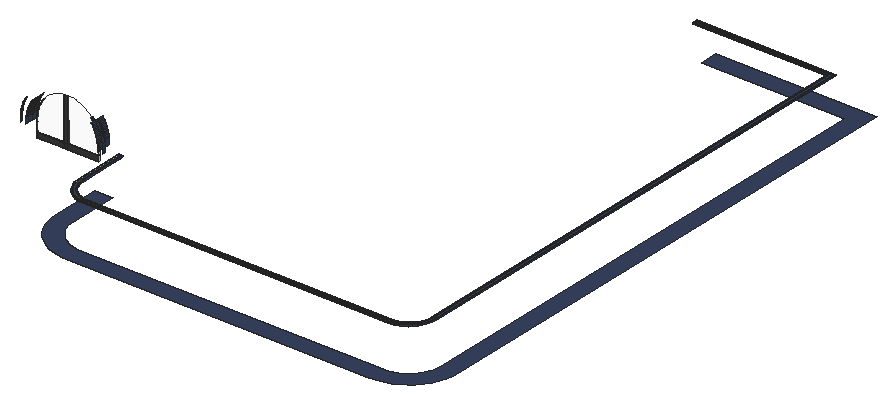
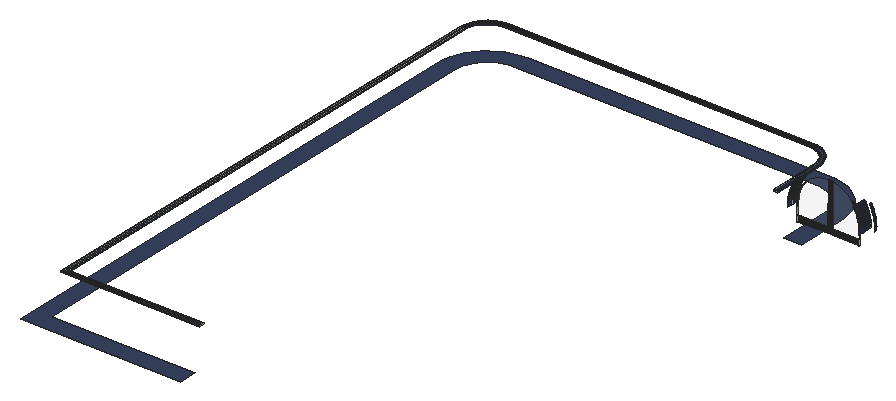
# SketchUp Ruby script. Lengths in inches.
U = 1.inch
M = Sketchup.active_model
def pt(a) = Geom::Point3d.new(a.map { |v| v * U })
def face(e, loops, mat)
  f = e.add_face(loops[0].map { |a| pt(a) })
  loops[1..].each { |l| e.add_face(l.map { |a| pt(a) }).erase! }
  f.material = f.back_material = mat if mat
  f
end
# faces: each face lists its corners as indices into pts; further lists are holes
def faces(e, pts, list, mat = nil) = list.each { |f| face(e, (f[0].is_a?(Array) ? f : [f]).map { |l| l.map { |i| pts[i] } }, mat) }
# xy, xz, yz: faces in a plane at the given z, y or x. An outline is a flat list of corners, or four numbers for a rectangle; further outlines are holes
def ring(l) = l.size == 4 ? [[l[0], l[1]], [l[2], l[1]], [l[2], l[3]], [l[0], l[3]]] : l.each_slice(2).to_a
def flat(e, list, mat, &to3) = list.each { |f| face(e, (f[0].is_a?(Array) ? f : [f]).map { |l| ring(l).map { |u, v| to3.(u, v) } }, mat) }
def xy(e, z, list, mat = nil) = flat(e, list, mat) { |x, y| [x, y, z] }
def xz(e, y, list, mat = nil) = flat(e, list, mat) { |x, z| [x, y, z] }
def yz(e, x, list, mat = nil) = flat(e, list, mat) { |y, z| [x, y, z] }
def lines(e, pts, list) = list.each { |a, b| e.add_line(pt(pts[a]), pt(pts[b])) }
# prism: a flat outline (further loops are holes) pulled along v
def prism(e, loops, v, mat = nil)
  f = face(e, loops, mat); d = Geom::Vector3d.new(v.map { |x| x * U })
  f.pushpull(f.normal.samedirection?(d) ? d.length : -d.length)
end
def box(e, o, s, mat = nil) = prism(e, [[o, [o[0] + s[0], o[1], o[2]], [o[0] + s[0], o[1] + s[1], o[2]], [o[0], o[1] + s[1], o[2]]]], [0, 0, s[2]], mat)
def at(x, y, z, deg = 0) = Geom::Transformation.translation(pt([x, y, z])) * Geom::Transformation.rotation(ORIGIN, Z_AXIS, deg.degrees)
def axes(o, x, y, z) = Geom::Transformation.new([*x, 0, *y, 0, *z, 0, *pt(o).to_a, 1])
def part(name) = M.definitions.add(name)
# library, detail: a bought-in or finely detailed component or shape, given as its bounding box
def library(name, o, s) = part(name).tap { |d| box(d.entities, o, s) }
def detail(e, o, s) = box(e.add_group.entities, o, s)
def put(e, d, t, mat = nil) = e.add_instance(d, t).tap { |i| i.material = mat if mat }
def group(e, t, mat = nil) = e.add_group.tap { |g| g.transformation = t; g.material = mat if mat }.entities
root = M.entities
M.materials.add("0360 AP 9644 Monsoon Midnight-N").color = [56, 67, 95]
M.materials.add("Glass Clear 001").color = [246, 246, 246]
M.materials["Glass Clear 001"].alpha = 0.1
M.materials.add("[Color M07]").color = [58, 58, 58]
xy(root,273.625,[[134.21,17.08,360,17.08,364.8125,17.39,369.54,18.34,374.11,19.88,378.43,22.02,382.4375,24.7,386.0625,27.875,389.24,31.5,391.92,35.51,394.05,39.83,395.6,44.4,396.54,49.125,396.86,53.9375,396.86,438.8,278.3125,438.8,278.3125,425.9375,384,425.9375,384,53.9375,383.79,50.8,383.18,47.73,382.17,44.75,380.78,41.9375,379.04,39.33,376.97,36.97,374.61,34.9,372,33.15,369.18,31.76,366.21,30.76,363.13,30.14,360,29.9375,134.95,29.9375,131.9375,30.29,128.99,31.02,126.8125,31.86,126.15,32.11,123.48,33.56,121.01,35.33,118.78,37.4,116.84,39.73,115.2,42.29,113.9,45.03,112.95,47.92,112.38,50.91,112.1875,53.9375,112.1875,89.9375,99.33,89.9375,99.33,53.53,99.6,49.28,100.48,44.7,101.93,40.26,103.93,36.04,106.45,32.11,109.4375,28.53,112.86,25.35,116.65,22.63,120.76,20.42,122.17,19.87,125.11,18.73,129.64,17.61]],"0360 AP 9644 Monsoon Midnight-N")
xy(root,291.19,[[53.24,93.58,73.03,94.27],[76.4,93.58,98.89,94.27]])
xy(root,294.87,[[53.24,93.58,73.03,94.27],[76.36,93.58,98.89,94.27]],"[Color M07]")
xy(root,302.6875,[[135.22,34.55,132.76,34.83,130.375,35.42,128.47,36.16,128.09,36.31,125.93,37.47,123.93,38.9,122.13,40.57,120.5625,42.46,119.24,44.53,118.1875,46.74,117.42,49.08,116.96,51.49,116.8,54.08,116.8,89.9375,118.94,89.9375,118.94,54.15,119.09,51.76,119.5,49.62,120.18,47.54,121.12,45.57,122.29,43.73,123.69,42.05,125.29,40.57,127.07,39.3,128.99,38.26,129.25,38.16,131.02,37.47,133.14,36.95,135.35,36.69,360,36.69,362.25,36.84,364.46,37.28,366.6,38,368.625,39,370.5,40.25,372.2,41.74,373.68,43.4375,374.9375,45.3125,375.93,47.34,376.66,49.47,377.1,51.6875,377.25,53.9375,377.25,419.18,278.3125,419.18,278.3125,421.33,379.39,421.33,379.39,53.9375,379.23,51.41,378.73,48.92,377.92,46.52,376.79,44.24,375.39,42.13,373.71,40.23,371.81,38.55,369.7,37.14,367.42,36.02,365.02,35.21,362.53,34.71,360,34.55]])
xy(root,302.6875,[[[135.18,33.89,132.64,34.18,130.18,34.79,128.24,35.54,127.8125,35.71,125.58,36.92,123.52,38.39,121.66,40.12,120.03,42.07,118.66,44.21,117.58,46.5,116.79,48.91,116.31,51.4,116.14,54.0625,116.14,90.59,119.6,90.59,119.6,54.17,119.74,51.84,120.14,49.78,120.79,47.78,121.69,45.89,122.83,44.12,124.17,42.51,125.71,41.08,127.42,39.85,129.26,38.86,129.48,38.77,131.22,38.1,133.26,37.59,135.38,37.35,360,37.35,362.17,37.49,364.29,37.91,366.35,38.61,368.3,39.57,370.1,40.78,371.73,42.21,373.16,43.84,374.37,45.64,375.33,47.59,376.03,49.64,376.45,51.77,376.59,53.9375,376.59,418.53,277.66,418.53,277.66,421.99,380.05,421.99,380.05,53.9375,379.88,51.32,379.37,48.75,378.52,46.27,377.36,43.91,375.91,41.73,374.18,39.76,372.2,38.03,370.02,36.57,367.67,35.42,365.1875,34.57,362.62,34.06,360,33.89],[135.22,34.55,360,34.55,362.53,34.71,365.02,35.21,367.42,36.02,369.7,37.14,371.81,38.55,373.71,40.23,375.39,42.13,376.79,44.24,377.92,46.52,378.73,48.92,379.23,51.41,379.39,53.9375,379.39,421.33,278.3125,421.33,278.3125,419.18,377.25,419.18,377.25,53.9375,377.1,51.6875,376.66,49.47,375.93,47.34,374.9375,45.3125,373.68,43.4375,372.2,41.74,370.5,40.25,368.625,39,366.6,38,364.46,37.28,362.25,36.84,360,36.69,135.35,36.69,133.14,36.95,131.02,37.47,129.25,38.16,128.99,38.26,127.07,39.3,125.29,40.57,123.69,42.05,122.29,43.73,121.12,45.57,120.18,47.54,119.5,49.62,119.09,51.76,118.94,54.15,118.94,89.9375,116.8,89.9375,116.8,54.08,116.96,51.49,117.42,49.08,118.1875,46.74,119.24,44.53,120.5625,42.46,122.13,40.57,123.93,38.9,125.93,37.47,128.09,36.31,128.47,36.16,130.375,35.42,132.76,34.83]]],"0360 AP 9644 Monsoon Midnight-N")
xy(root,303.4375,[[[135.18,33.89,360,33.89,362.62,34.06,365.1875,34.57,367.67,35.42,370.02,36.57,372.2,38.03,374.18,39.76,375.91,41.73,377.36,43.91,378.52,46.27,379.37,48.75,379.88,51.32,380.05,53.9375,380.05,421.99,277.66,421.99,277.66,418.53,376.59,418.53,376.59,53.9375,376.45,51.77,376.03,49.64,375.33,47.59,374.37,45.64,373.16,43.84,371.73,42.21,370.1,40.78,368.3,39.57,366.35,38.61,364.29,37.91,362.17,37.49,360,37.35,135.38,37.35,133.26,37.59,131.22,38.1,129.48,38.77,129.26,38.86,127.42,39.85,125.71,41.08,124.17,42.51,122.83,44.12,121.69,45.89,120.79,47.78,120.14,49.78,119.74,51.84,119.6,54.17,119.6,90.59,116.14,90.59,116.14,54.0625,116.31,51.4,116.79,48.91,117.58,46.5,118.66,44.21,120.03,42.07,121.66,40.12,123.52,38.39,125.58,36.92,127.8125,35.71,128.24,35.54,130.18,34.79,132.64,34.18],[135.22,34.55,132.76,34.83,130.375,35.42,128.47,36.16,128.09,36.31,125.93,37.47,123.93,38.9,122.13,40.57,120.5625,42.46,119.24,44.53,118.1875,46.74,117.42,49.08,116.96,51.49,116.8,54.08,116.8,89.9375,118.94,89.9375,118.94,54.15,119.09,51.76,119.5,49.62,120.18,47.54,121.12,45.57,122.29,43.73,123.69,42.05,125.29,40.57,127.07,39.3,128.99,38.26,129.25,38.16,131.02,37.47,133.14,36.95,135.35,36.69,360,36.69,362.25,36.84,364.46,37.28,366.6,38,368.625,39,370.5,40.25,372.2,41.74,373.68,43.4375,374.9375,45.3125,375.93,47.34,376.66,49.47,377.1,51.6875,377.25,53.9375,377.25,419.18,278.3125,419.18,278.3125,421.33,379.39,421.33,379.39,53.9375,379.23,51.41,378.73,48.92,377.92,46.52,376.79,44.24,375.39,42.13,373.71,40.23,371.81,38.55,369.7,37.14,367.42,36.02,365.02,35.21,362.53,34.71,360,34.55]],[135.22,34.55,360,34.55,362.53,34.71,365.02,35.21,367.42,36.02,369.7,37.14,371.81,38.55,373.71,40.23,375.39,42.13,376.79,44.24,377.92,46.52,378.73,48.92,379.23,51.41,379.39,53.9375,379.39,421.33,278.3125,421.33,278.3125,419.18,377.25,419.18,377.25,53.9375,377.1,51.6875,376.66,49.47,375.93,47.34,374.9375,45.3125,373.68,43.4375,372.2,41.74,370.5,40.25,368.625,39,366.6,38,364.46,37.28,362.25,36.84,360,36.69,135.35,36.69,133.14,36.95,131.02,37.47,129.25,38.16,128.99,38.26,127.07,39.3,125.29,40.57,123.69,42.05,122.29,43.73,121.12,45.57,120.18,47.54,119.5,49.62,119.09,51.76,118.94,54.15,118.94,89.9375,116.8,89.9375,116.8,54.08,116.96,51.49,117.42,49.08,118.1875,46.74,119.24,44.53,120.5625,42.46,122.13,40.57,123.93,38.9,125.93,37.47,128.09,36.31,128.47,36.16,130.375,35.42,132.76,34.83]],"0360 AP 9644 Monsoon Midnight-N")
xz(root,33.89,[[135.18,302.6875,360,303.4375]],"0360 AP 9644 Monsoon Midnight-N")
xz(root,34.55,[[135.22,302.6875,360,303.4375]])
xz(root,36.69,[[135.35,302.6875,360,303.4375]])
xz(root,37.35,[[135.38,302.6875,360,303.4375]],"0360 AP 9644 Monsoon Midnight-N")
xz(root,89.9375,[[49.72,301.29,49.72,305.77,49.71,305.66,49.65,304.79,49.625,303.91,49.63,303.04,49.66,302.16],[102.41,301.29,102.47,302.16,102.5,303.04,102.5,303.91,102.47,304.79,102.42,305.66,102.41,305.77],[116.8,302.6875,117.8125,303.4375],[117.8125,302.6875,118.94,303.4375]])
xz(root,90.59,[[116.14,302.6875,117.8125,303.4375],[117.8125,302.6875,119.6,303.4375]])
xz(root,93.58,[[53.24,291.19,73.03,294.87],[73.03,291.19,76.4,291.19,76.36,294.87,73.03,294.87],[76.4,291.19,98.89,291.19,98.89,294.87,76.36,294.87],[73.03,294.87,76.36,294.87,76.0625,326.46,75.3,326.45,74.55,326.41,73.79,326.35,73.03,326.26]],"[Color M07]")
xz(root,94.27,[[53.24,294.87,73.03,294.87,73.03,326.26,72.28,326.15,71.54,326.01,70.8,325.85,70.06,325.66,69.33,325.45,68.61,325.21,67.9,324.95,67.19,324.67,66.5,324.37,65.8125,324.04,65.14,323.6875,64.48,323.32,63.83,322.92,63.19,322.51,62.57,322.07,61.97,321.61,61.375,321.13,60.8,320.64,60.24,320.125,59.7,319.59,59.18,319.04,58.67,318.47,58.19,317.89,57.72,317.29,57.28,316.67,56.85,316.05,56.45,315.4,56.07,314.75,55.71,314.08,55.37,313.4,55.06,312.71,54.76,312.01,54.49,311.3,54.25,310.58,54.03,309.85,53.83,309.12,53.66,308.38,53.51,307.64,53.39,306.89,53.29,306.13,53.24,305.6],[76.36,294.87,98.89,294.87,98.89,305.6,98.84,306.13,98.74,306.89,98.62,307.64,98.47,308.38,98.29,309.12,98.1,309.85,97.875,310.58,97.63,311.3,97.36,312.01,97.07,312.71,96.75,313.4,96.42,314.08,96.06,314.75,95.67,315.4,95.27,316.05,94.85,316.67,94.4,317.29,93.94,317.89,93.45,318.47,92.95,319.04,92.42,319.59,91.88,320.125,91.32,320.64,90.75,321.13,90.16,321.61,89.55,322.07,88.93,322.51,88.3,322.92,87.65,323.32,86.99,323.6875,86.3125,324.04,85.63,324.37,84.93,324.67,84.23,324.95,83.52,325.21,82.79,325.45,82.06,325.66,81.33,325.85,80.59,326.01,79.84,326.15,79.09,326.26,78.34,326.35,77.58,326.41,76.82,326.45,76.0625,326.46]],"Glass Clear 001")
xz(root,418.53,[[277.66,302.6875,376.59,303.4375]])
xz(root,419.18,[[278.3125,302.6875,377.25,303.4375]])
xz(root,421.33,[[278.3125,302.6875,379.39,303.4375]])
xz(root,421.99,[[277.66,302.6875,380.05,303.4375]])
yz(root,49.72,[[88.375,301.29,89.9375,305.77],[89.9375,301.29,93.58,305.77],[94.96,301.29,98.79,305.77]],"0360 AP 9644 Monsoon Midnight-N")
yz(root,49.72,[[93.58,301.29,94.96,305.77]],"[Color M07]")
yz(root,53.24,[[93.58,291.19,94.96,294.87]])
yz(root,53.24,[[93.58,294.87,94.27,301.29],[93.58,301.29,94.27,305.6]],"[Color M07]")
yz(root,73.03,[[93.58,294.87,94.27,326.26]],"[Color M07]")
yz(root,98.89,[[93.58,291.19,94.96,294.87],[94.27,294.87,94.96,301.29],[94.27,301.29,94.96,305.6]])
yz(root,98.89,[[93.58,294.87,94.27,301.29],[93.58,301.29,94.27,305.6]],"[Color M07]")
yz(root,102.41,[[93.58,301.29,94.96,305.77]])
yz(root,102.41,[[88.375,301.29,89.9375,305.77],[89.9375,301.29,93.58,305.77],[94.96,301.29,98.79,305.77]],"0360 AP 9644 Monsoon Midnight-N")
yz(root,102.5,[[88.375,303.04,89.9375,303.91]])
yz(root,116.14,[[54.0625,302.6875,90.59,303.4375]],"0360 AP 9644 Monsoon Midnight-N")
yz(root,116.8,[[54.08,302.6875,89.9375,303.4375]])
yz(root,118.94,[[54.15,302.6875,89.9375,303.4375]])
yz(root,119.6,[[54.17,302.6875,90.59,303.4375]],"0360 AP 9644 Monsoon Midnight-N")
yz(root,277.66,[[418.53,302.6875,421.99,303.4375]])
yz(root,278.3125,[[419.18,302.6875,421.33,303.4375]])
yz(root,376.59,[[53.9375,302.6875,418.53,303.4375]],"0360 AP 9644 Monsoon Midnight-N")
yz(root,377.25,[[53.9375,302.6875,419.18,303.4375]])
yz(root,379.39,[[53.9375,302.6875,421.33,303.4375]])
yz(root,380.05,[[53.9375,302.6875,421.99,303.4375]],"0360 AP 9644 Monsoon Midnight-N")
p = [[76.36,94.27,294.87],[76.0625,94.27,326.46],[76.0625,93.58,326.46],[76.36,93.58,294.87],[45.48,89.9375,301.94],[45.54,89.9375,301.15],
  [45.54,88.375,301.15],[45.48,88.375,301.94],[106.59,89.9375,301.15],[106.64,89.9375,301.94],[106.64,88.375,301.94],[106.59,88.375,301.15],
  [49.72,89.9375,301.29],[49.66,89.9375,302.16],[49.66,88.375,302.16],[49.72,88.375,301.29],[102.47,89.9375,302.16],[102.41,89.9375,301.29],
  [102.41,88.375,301.29],[102.47,88.375,302.16],[45.45,89.9375,302.96],[45.45,88.375,302.96],[106.63,89.9375,304.01],[106.63,88.375,304.01],
  [49.63,89.9375,303.04],[49.63,88.375,303.04],[102.5,89.9375,303.04],[102.5,88.375,303.04],[132.64,34.18,302.6875],[135.18,33.89,302.6875],
  [135.18,33.89,303.4375],[132.64,34.18,303.4375],[360,33.89,302.6875],[362.62,34.06,302.6875],[362.62,34.06,303.4375],[360,33.89,303.4375],
  [365.1875,34.57,302.6875],[365.1875,34.57,303.4375],[130.18,34.79,302.6875],[130.18,34.79,303.4375],[135.22,34.55,302.6875],[132.76,34.83,302.6875],
  [132.76,34.83,303.4375],[135.22,34.55,303.4375],[362.53,34.71,302.6875],[360,34.55,302.6875],[360,34.55,303.4375],[362.53,34.71,303.4375],
  [367.67,35.42,302.6875],[367.67,35.42,303.4375],[365.02,35.21,302.6875],[365.02,35.21,303.4375],[128.24,35.54,302.6875],[128.24,35.54,303.4375],
  [130.375,35.42,302.6875],[130.375,35.42,303.4375],[367.42,36.02,302.6875],[367.42,36.02,303.4375],[128.47,36.16,302.6875],[128.47,36.16,303.4375],
  [370.02,36.57,302.6875],[370.02,36.57,303.4375],[127.8125,35.71,302.6875],[127.8125,35.71,303.4375],[125.58,36.92,302.6875],[125.58,36.92,303.4375],
  [369.7,37.14,302.6875],[369.7,37.14,303.4375],[128.09,36.31,302.6875],[128.09,36.31,303.4375],[125.93,37.47,302.6875],[125.93,37.47,303.4375],
  [372.2,38.03,302.6875],[372.2,38.03,303.4375],[133.14,36.95,302.6875],[135.35,36.69,302.6875],[135.35,36.69,303.4375],[133.14,36.95,303.4375],
  [360,36.69,302.6875],[362.25,36.84,302.6875],[362.25,36.84,303.4375],[360,36.69,303.4375],[364.46,37.28,302.6875],[364.46,37.28,303.4375],
  [123.52,38.39,302.6875],[123.52,38.39,303.4375],[131.02,37.47,302.6875],[131.02,37.47,303.4375],[371.81,38.55,302.6875],[371.81,38.55,303.4375],
  [135.38,37.35,302.6875],[133.26,37.59,302.6875],[133.26,37.59,303.4375],[135.38,37.35,303.4375],[362.17,37.49,302.6875],[360,37.35,302.6875],
  [360,37.35,303.4375],[362.17,37.49,303.4375],[366.6,38,302.6875],[366.6,38,303.4375],[123.93,38.9,302.6875],[123.93,38.9,303.4375],
  [129.25,38.16,302.6875],[129.25,38.16,303.4375],[364.29,37.91,302.6875],[364.29,37.91,303.4375],[131.22,38.1,302.6875],[131.22,38.1,303.4375],
  [366.35,38.61,302.6875],[366.35,38.61,303.4375],[368.625,39,302.6875],[368.625,39,303.4375],[374.18,39.76,302.6875],[374.18,39.76,303.4375],
  [129.48,38.77,302.6875],[129.48,38.77,303.4375],[128.99,38.26,302.6875],[128.99,38.26,303.4375],[127.07,39.3,302.6875],[127.07,39.3,303.4375],
  [121.66,40.12,302.6875],[121.66,40.12,303.4375],[368.3,39.57,302.6875],[368.3,39.57,303.4375],[373.71,40.23,302.6875],[373.71,40.23,303.4375],
  [129.26,38.86,302.6875],[129.26,38.86,303.4375],[122.13,40.57,302.6875],[122.13,40.57,303.4375],[127.42,39.85,302.6875],[127.42,39.85,303.4375],
  [370.5,40.25,302.6875],[370.5,40.25,303.4375],[125.29,40.57,302.6875],[125.29,40.57,303.4375],[370.1,40.78,302.6875],[370.1,40.78,303.4375],
  [375.91,41.73,302.6875],[375.91,41.73,303.4375],[125.71,41.08,302.6875],[125.71,41.08,303.4375],[120.03,42.07,302.6875],[120.03,42.07,303.4375],
  [375.39,42.13,302.6875],[375.39,42.13,303.4375],[372.2,41.74,302.6875],[372.2,41.74,303.4375],[120.5625,42.46,302.6875],[120.5625,42.46,303.4375],
  [123.69,42.05,302.6875],[123.69,42.05,303.4375],[371.73,42.21,302.6875],[371.73,42.21,303.4375],[124.17,42.51,302.6875],[124.17,42.51,303.4375],
  [373.68,43.4375,302.6875],[373.68,43.4375,303.4375],[377.36,43.91,302.6875],[377.36,43.91,303.4375],[118.66,44.21,302.6875],[118.66,44.21,303.4375],
  [122.29,43.73,302.6875],[122.29,43.73,303.4375],[376.79,44.24,302.6875],[376.79,44.24,303.4375],[373.16,43.84,302.6875],[373.16,43.84,303.4375],
  [119.24,44.53,302.6875],[119.24,44.53,303.4375],[122.83,44.12,302.6875],[122.83,44.12,303.4375],[374.9375,45.3125,302.6875],[374.9375,45.3125,303.4375],
  [121.12,45.57,302.6875],[121.12,45.57,303.4375],[374.37,45.64,302.6875],[374.37,45.64,303.4375],[378.52,46.27,302.6875],[378.52,46.27,303.4375],
  [121.69,45.89,302.6875],[121.69,45.89,303.4375],[117.58,46.5,302.6875],[117.58,46.5,303.4375],[377.92,46.52,302.6875],[377.92,46.52,303.4375],
  [118.1875,46.74,302.6875],[118.1875,46.74,303.4375],[375.93,47.34,302.6875],[375.93,47.34,303.4375],[120.18,47.54,302.6875],[120.18,47.54,303.4375],
  [375.33,47.59,302.6875],[375.33,47.59,303.4375],[120.79,47.78,302.6875],[120.79,47.78,303.4375],[379.37,48.75,302.6875],[379.37,48.75,303.4375],
  [116.79,48.91,302.6875],[116.79,48.91,303.4375],[378.73,48.92,302.6875],[378.73,48.92,303.4375],[117.42,49.08,302.6875],[117.42,49.08,303.4375],
  [376.66,49.47,302.6875],[376.66,49.47,303.4375],[119.5,49.62,302.6875],[119.5,49.62,303.4375],[376.03,49.64,302.6875],[376.03,49.64,303.4375],
  [120.14,49.78,302.6875],[120.14,49.78,303.4375],[379.88,51.32,302.6875],[379.88,51.32,303.4375],[116.31,51.4,302.6875],[116.31,51.4,303.4375],
  [379.23,51.41,302.6875],[379.23,51.41,303.4375],[116.96,51.49,302.6875],[116.96,51.49,303.4375],[377.1,51.6875,302.6875],[377.1,51.6875,303.4375],
  [119.09,51.76,302.6875],[119.09,51.76,303.4375],[376.45,51.77,302.6875],[376.45,51.77,303.4375],[119.74,51.84,302.6875],[119.74,51.84,303.4375],
  [380.05,53.9375,302.6875],[380.05,53.9375,303.4375],[116.14,54.0625,302.6875],[116.14,54.0625,303.4375],[379.39,53.9375,302.6875],[379.39,53.9375,303.4375],
  [116.8,54.08,302.6875],[116.8,54.08,303.4375],[377.25,53.9375,302.6875],[377.25,53.9375,303.4375],[118.94,54.15,302.6875],[118.94,54.15,303.4375],
  [119.6,54.17,302.6875],[119.6,54.17,303.4375],[376.59,53.9375,302.6875],[376.59,53.9375,303.4375],[45.44,89.9375,303.97],[45.44,88.375,303.97],
  [49.625,89.9375,303.91],[49.625,88.375,303.91],[49.65,89.9375,304.79],[49.65,88.375,304.79],[102.47,89.9375,304.79],[102.5,89.9375,303.91],
  [102.5,88.375,303.91],[102.47,88.375,304.79],[45.48,89.9375,304.99],[45.48,88.375,304.99],[106.49,89.9375,306.08],[106.49,88.375,306.08],
  [49.71,89.9375,305.66],[49.71,88.375,305.66],[102.42,89.9375,305.66],[102.42,88.375,305.66],[45.54,89.9375,306],[45.54,88.375,306],
  [53.24,94.27,305.6],[53.29,94.27,306.13],[53.29,93.58,306.13],[53.24,93.58,305.6],[98.84,94.27,306.13],[98.89,94.27,305.6],
  [98.89,93.58,305.6],[98.84,93.58,306.13],[98.84,94.96,306.13],[98.89,94.96,305.6],[49.72,89.9375,305.77],[49.72,88.375,305.77],
  [102.41,89.9375,305.77],[102.41,88.375,305.77],[49.72,93.58,305.77],[49.79,93.58,306.53],[49.79,88.375,306.53],[102.33,88.375,306.53],
  [102.33,93.58,306.53],[102.41,93.58,305.77],[49.79,94.96,306.53],[49.72,94.96,305.77],[102.41,94.96,305.77],[102.33,94.96,306.53],
  [49.79,98.79,306.53],[49.72,98.79,305.77],[102.41,98.79,305.77],[102.33,98.79,306.53],[45.56,89.9375,306.17],[45.56,88.375,306.17],
  [106.22,89.9375,308.125],[106.22,88.375,308.125],[53.39,94.27,306.89],[53.39,93.58,306.89],[98.74,94.27,306.89],[98.74,93.58,306.89],
  [98.74,94.96,306.89],[45.64,89.9375,307.01],[45.64,88.375,307.01],[49.91,93.58,307.4],[49.91,88.375,307.4],[102.22,88.375,307.4],
  [102.22,93.58,307.4],[49.91,94.96,307.4],[102.22,94.96,307.4],[49.91,98.79,307.4],[102.22,98.79,307.4],[53.51,94.27,307.64],
  [53.51,93.58,307.64],[98.62,94.27,307.64],[98.62,93.58,307.64],[98.62,94.96,307.64],[45.77,89.9375,308.01],[45.77,88.375,308.01],
  [50.05,93.58,308.27],[50.05,88.375,308.27],[102.08,88.375,308.27],[102.08,93.58,308.27],[50.05,94.96,308.27],[102.08,94.96,308.27],
  [50.05,98.79,308.27],[102.08,98.79,308.27],[53.66,94.27,308.38],[53.66,93.58,308.38],[98.47,94.27,308.38],[98.47,93.58,308.38],
  [98.47,94.96,308.38],[45.94,89.9375,309.01],[45.94,88.375,309.01],[105.8125,89.9375,310.15],[105.8125,88.375,310.15],[50.22,93.58,309.125],
  [50.22,88.375,309.125],[101.9,88.375,309.125],[101.9,93.58,309.125],[50.22,94.96,309.125],[101.9,94.96,309.125],[50.22,98.79,309.125],
  [101.9,98.79,309.125],[53.83,94.27,309.12],[53.83,93.58,309.12],[98.29,94.27,309.12],[98.29,93.58,309.12],[98.29,94.96,309.12],
  [46.13,89.9375,310.01],[46.13,88.375,310.01],[50.42,93.58,309.98],[50.42,88.375,309.98],[101.71,88.375,309.98],[101.71,93.58,309.98],
  [50.42,94.96,309.98],[54.03,94.27,309.85],[54.03,93.58,309.85],[98.1,94.27,309.85],[98.1,93.58,309.85],[101.71,94.96,309.98],
  [98.1,94.96,309.85],[50.42,98.79,309.98],[101.71,98.79,309.98],[54.25,94.27,310.58],[54.25,93.58,310.58],[97.875,94.27,310.58],
  [97.875,93.58,310.58],[97.875,94.96,310.58],[46.36,89.9375,311],[46.36,88.375,311],[50.65,93.58,310.82],[50.65,88.375,310.82],
  [101.48,88.375,310.82],[101.48,93.58,310.82],[50.65,94.96,310.82],[101.48,94.96,310.82],[50.65,98.79,310.82],[101.48,98.79,310.82],
  [105.28,89.9375,312.15],[105.28,88.375,312.15],[54.49,94.27,311.3],[54.49,93.58,311.3],[97.63,94.27,311.3],[97.63,93.58,311.3],
  [97.63,94.96,311.3],[50.9,93.58,311.66],[50.9,88.375,311.66],[101.22,88.375,311.66],[101.22,93.58,311.66],[50.9,94.96,311.66],
  [101.22,94.96,311.66],[50.9,98.79,311.66],[101.22,98.79,311.66],[46.63,89.9375,311.97],[46.63,88.375,311.97],[54.76,94.27,312.01],
  [54.76,93.58,312.01],[97.36,94.27,312.01],[97.36,93.58,312.01],[97.36,94.96,312.01],[51.18,93.58,312.49],[51.18,88.375,312.49],
  [100.94,88.375,312.49],[100.94,93.58,312.49],[51.18,94.96,312.49],[100.94,94.96,312.49],[51.18,98.79,312.49],[100.94,98.79,312.49],
  [46.92,89.9375,312.94],[46.92,88.375,312.94],[55.06,94.27,312.71],[55.06,93.58,312.71],[97.07,94.27,312.71],[97.07,93.58,312.71],
  [97.07,94.96,312.71],[104.625,89.9375,314.11],[104.625,88.375,314.11],[51.49,93.58,313.31],[51.49,88.375,313.31],[100.63,88.375,313.31],
  [100.63,93.58,313.31],[51.49,94.96,313.31],[100.63,94.96,313.31],[51.49,98.79,313.31],[100.63,98.79,313.31],[55.37,94.27,313.4],
  [55.37,93.58,313.4],[96.75,94.27,313.4],[96.75,93.58,313.4],[96.75,94.96,313.4],[47.25,89.9375,313.9],[47.25,88.375,313.9],
  [51.83,93.58,314.12],[51.83,88.375,314.12],[100.29,88.375,314.12],[100.29,93.58,314.12],[51.83,94.96,314.12],[100.29,94.96,314.12],
  [51.83,98.79,314.12],[100.29,98.79,314.12],[55.71,94.27,314.08],[55.71,93.58,314.08],[96.42,94.27,314.08],[96.42,93.58,314.08],
  [96.42,94.96,314.08],[47.61,89.9375,314.85],[47.61,88.375,314.85],[52.2,93.58,314.91],[52.2,88.375,314.91],[99.93,88.375,314.91],
  [99.93,93.58,314.91],[103.85,89.9375,316.03],[103.85,88.375,316.03],[52.2,94.96,314.91],[56.07,94.27,314.75],[56.07,93.58,314.75],
  [96.06,94.27,314.75],[96.06,93.58,314.75],[99.93,94.96,314.91],[96.06,94.96,314.75],[52.2,98.79,314.91],[99.93,98.79,314.91],
  [56.45,94.27,315.4],[56.45,93.58,315.4],[95.67,94.27,315.4],[95.67,93.58,315.4],[95.67,94.96,315.4],[48,89.9375,315.79],
  [48,88.375,315.79],[52.59,93.58,315.7],[52.59,88.375,315.7],[99.54,88.375,315.7],[99.54,93.58,315.7],[52.59,94.96,315.7],
  [99.54,94.96,315.7],[52.59,98.79,315.7],[99.54,98.79,315.7],[56.85,94.27,316.05],[56.85,93.58,316.05],[95.27,94.27,316.05],
  [95.27,93.58,316.05],[95.27,94.96,316.05],[53,93.58,316.47],[53,88.375,316.47],[99.125,88.375,316.47],[99.125,93.58,316.47],
  [53,94.96,316.47],[99.125,94.96,316.47],[53,98.79,316.47],[99.125,98.79,316.47],[48.42,89.9375,316.71],[48.42,88.375,316.71],
  [102.95,89.9375,317.89],[102.95,88.375,317.89],[57.28,94.27,316.67],[57.28,93.58,316.67],[94.85,94.27,316.67],[94.85,93.58,316.67],
  [94.85,94.96,316.67],[53.44,93.58,317.22],[53.44,88.375,317.22],[98.68,88.375,317.22],[98.68,93.58,317.22],[53.44,94.96,317.22],
  [98.68,94.96,317.22],[53.44,98.79,317.22],[98.68,98.79,317.22],[48.87,89.9375,317.62],[48.87,88.375,317.62],[57.72,94.27,317.29],
  [57.72,93.58,317.29],[94.4,94.27,317.29],[94.4,93.58,317.29],[94.4,94.96,317.29],[53.91,93.58,317.96],[53.91,88.375,317.96],
  [98.22,88.375,317.96],[98.22,93.58,317.96],[53.91,94.96,317.96],[98.22,94.96,317.96],[53.91,98.79,317.96],[98.22,98.79,317.96],
  [58.19,94.27,317.89],[58.19,93.58,317.89],[93.94,94.27,317.89],[93.94,93.58,317.89],[93.94,94.96,317.89],[49.35,89.9375,318.51],
  [49.35,88.375,318.51],[101.93,89.9375,319.69],[101.93,88.375,319.69],[58.67,94.27,318.47],[58.67,93.58,318.47],[93.45,94.27,318.47],
  [93.45,93.58,318.47],[93.45,94.96,318.47],[54.4,93.58,318.69],[54.4,88.375,318.69],[97.73,88.375,318.69],[97.73,93.58,318.69],
  [54.4,94.96,318.69],[97.73,94.96,318.69],[54.4,98.79,318.69],[97.73,98.79,318.69],[58.19,94.96,317.89],[57.72,94.96,317.29],
  [57.28,94.96,316.67],[56.85,94.96,316.05],[56.45,94.96,315.4],[56.07,94.96,314.75],[55.71,94.96,314.08],[55.37,94.96,313.4],
  [55.06,94.96,312.71],[54.76,94.96,312.01],[54.49,94.96,311.3],[54.25,94.96,310.58],[54.03,94.96,309.85],[53.83,94.96,309.12],
  [53.66,94.96,308.38],[53.51,94.96,307.64],[53.39,94.96,306.89],[53.29,94.96,306.13],[53.24,94.96,305.6],[53.24,94.96,301.29],
  [53.24,94.27,301.29]]
faces(root,p,[[0,1,2,3],[28,29,30,31],[38,28,31,39],[52,38,39,53],[264,265,266,267],[268,269,270,271],[284,285,278,279],[286,287,282,283],
  [265,296,297,266],[298,268,271,299],[307,284,279,303],[287,308,306,282],[296,311,312,297],[313,298,299,314],[322,307,303,318],[308,323,321,306],
  [311,326,327,312],[328,313,314,329],[339,322,318,335],[323,340,338,321],[326,343,344,327],[345,328,329,346],[354,339,335,350],[343,355,356,344],
  [357,345,346,358],[340,359,353,338],[355,363,364,356],[365,357,358,366],[374,354,350,370],[359,375,373,353],[363,380,381,364],[382,365,366,383],
  [389,374,370,385],[375,390,388,373],[380,395,396,381],[397,382,383,398],[404,389,385,400],[390,405,403,388],[395,410,411,396],[412,397,398,413],
  [421,404,400,417],[405,422,420,403],[410,425,426,411],[427,412,413,428],[436,421,417,432],[422,437,435,420],[425,440,441,426],[442,427,428,443],
  [453,436,432,447],[440,454,455,441],[456,442,443,457],[437,458,450,435],[454,462,463,455],[464,456,457,465],[473,453,447,469],[458,474,472,450],
  [462,477,478,463],[479,464,465,480],[486,473,469,482],[474,487,485,472],[477,494,495,478],[496,479,480,497],[503,486,482,499],[487,504,502,485],
  [494,509,510,495],[511,496,497,512],[518,503,499,514],[504,519,517,502],[509,522,523,510],[524,511,512,525],[522,531,532,523],[533,524,525,534],
  [540,518,514,536],[519,541,539,517]],"[Color M07]")
faces(root,p,[[4,5,6,7],[8,9,10,11],[20,4,7,21],[9,22,23,10],[32,33,34,35],[33,36,37,34],[36,48,49,37],[48,60,61,49],
  [62,52,53,63],[64,62,63,65],[60,72,73,61],[84,64,65,85],[90,91,92,93],[94,95,96,97],[104,94,97,105],[91,106,107,92],
  [108,104,105,109],[72,112,113,73],[106,114,115,107],[120,84,85,121],[122,108,109,123],[114,126,127,115],[126,130,131,127],[136,122,123,137],
  [112,138,139,113],[130,140,141,131],[142,120,121,143],[152,136,137,153],[140,154,155,141],[138,158,159,139],[160,142,143,161],[166,152,153,167],
  [154,170,171,155],[176,166,167,177],[158,178,179,159],[170,180,181,171],[182,160,161,183],[192,176,177,193],[180,194,195,181],[178,196,197,179],
  [198,182,183,199],[208,192,193,209],[194,210,211,195],[196,212,213,197],[214,198,199,215],[224,208,209,225],[210,226,227,211],[212,228,229,213],
  [230,214,215,231],[226,240,241,227],[242,224,225,243],[244,20,21,245],[254,244,245,255],[22,256,257,23],[262,254,255,263],[274,278,279,280,275],
  [281,282,283,276,277],[288,284,285,289],[290,286,287,291],[292,262,263,293],[256,294,295,257],[301,292,293,302],[280,279,303,304],[305,306,282,281],
  [309,307,284,288],[291,287,308,310],[316,301,302,317],[304,303,318,319],[320,321,306,305],[324,322,307,309],[310,308,323,325],[331,316,317,332],
  [294,333,334,295],[319,318,335,336],[337,338,321,320],[341,339,322,324],[325,323,340,342],[348,331,332,349],[336,335,350,351],[352,353,338,337],
  [361,354,339,341],[342,340,359,362],[368,348,349,369],[351,350,370,371],[372,373,353,352],[376,374,354,361],[362,359,375,377],[333,378,379,334],
  [371,370,385,386],[387,388,373,372],[391,389,374,376],[377,375,390,392],[393,368,369,394],[386,385,400,401],[402,403,388,387],[406,404,389,391],
  [392,390,405,407],[408,393,394,409],[378,415,416,379],[401,400,417,418],[419,420,403,402],[423,421,404,406],[407,405,422,424],[430,408,409,431],
  [418,417,432,433],[434,435,420,419],[438,436,421,423],[424,422,437,439],[445,430,431,446],[433,432,447,448],[449,450,435,434],[415,451,452,416],
  [460,453,436,438],[439,437,458,461],[467,445,446,468],[448,447,469,470],[471,472,450,449],[475,473,453,460],[461,458,474,476],[470,469,482,483],
  [484,485,472,471],[488,486,473,475],[476,474,487,489],[490,467,468,491],[451,492,493,452],[483,482,499,500],[501,502,485,484],[505,503,486,488],
  [489,487,504,506],[507,490,491,508],[500,499,514,515],[516,517,502,501],[520,518,503,505],[506,504,519,521],[527,507,508,528],[492,529,530,493],
  [515,514,536,537],[538,539,517,516],[542,540,518,520],[521,519,541,543]],"0360 AP 9644 Monsoon Midnight-N")
faces(root,p,[[12,13,14,15],[16,17,18,19],[13,24,25,14],[26,16,19,27],[40,41,42,43],[44,45,46,47],[50,44,47,51],[41,54,55,42],
  [56,50,51,57],[54,58,59,55],[66,56,57,67],[58,68,69,59],[68,70,71,69],[74,75,76,77],[78,79,80,81],[79,82,83,80],
  [86,74,77,87],[88,66,67,89],[82,98,99,83],[70,100,101,71],[102,86,87,103],[98,110,111,99],[116,102,103,117],[118,116,117,119],
  [124,88,89,125],[100,128,129,101],[110,132,133,111],[134,118,119,135],[144,124,125,145],[132,146,147,133],[128,148,149,129],[150,134,135,151],
  [146,156,157,147],[162,150,151,163],[164,144,145,165],[148,168,169,149],[156,172,173,157],[174,162,163,175],[184,164,165,185],[168,186,187,169],
  [172,188,189,173],[190,174,175,191],[200,184,185,201],[186,202,203,187],[188,204,205,189],[206,190,191,207],[216,200,201,217],[202,218,219,203],
  [204,220,221,205],[222,206,207,223],[232,216,217,233],[218,234,235,219],[220,236,237,221],[238,222,223,239],[24,246,247,25],[246,248,249,247],
  [250,251,252,253],[248,258,259,249],[260,250,253,261],[272,273,269,268],[258,274,275,259],[276,260,261,277],[300,272,268,298],[315,300,298,313],
  [330,315,313,328],[347,330,328,345],[360,347,345,357],[367,360,357,365],[384,367,365,382],[399,384,382,397],[414,399,397,412],[429,414,412,427],
  [444,429,427,442],[459,444,442,456],[466,459,456,464],[481,466,464,479],[498,481,479,496],[513,498,496,511],[526,513,511,524],[535,526,524,533]])
lines(root,p,[[544,522],[545,509],[546,494],[547,477],[548,462],[549,454],[550,440],[551,425],[552,410],[553,395],[554,380],[555,363],
  [556,355],[557,343],[558,326],[559,311],[560,296],[561,265],[562,264],[563,564]])
